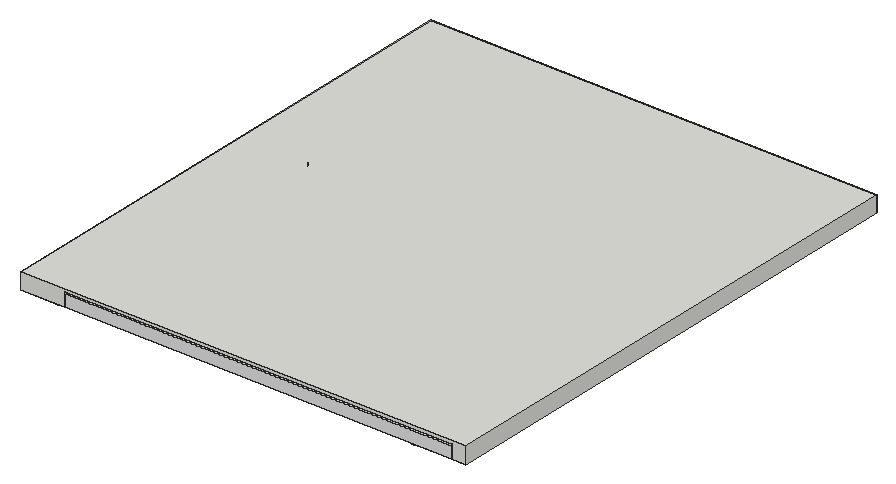
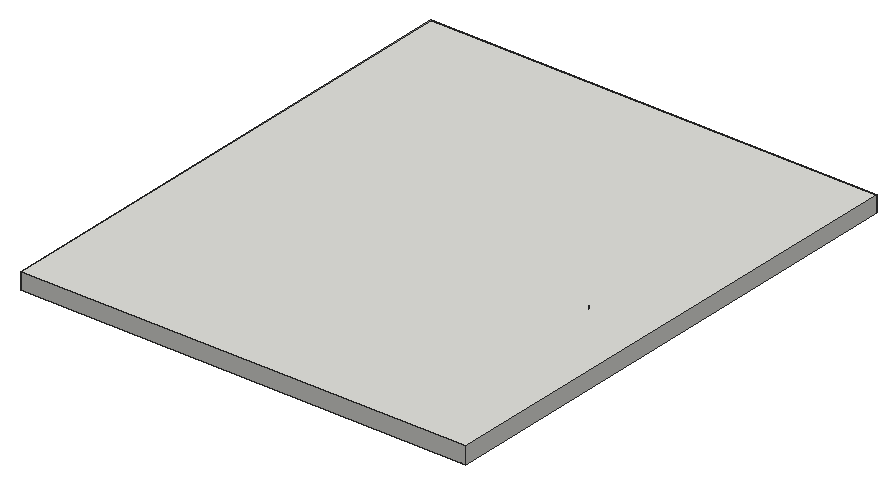
# SketchUp Ruby script. Lengths in inches.
U = 1.inch
M = Sketchup.active_model
def pt(a) = Geom::Point3d.new(a.map { |v| v * U })
def face(e, loops, mat)
  f = e.add_face(loops[0].map { |a| pt(a) })
  loops[1..].each { |l| e.add_face(l.map { |a| pt(a) }).erase! }
  f.material = f.back_material = mat if mat
  f
end
# faces: each face lists its corners as indices into pts; further lists are holes
def faces(e, pts, list, mat = nil) = list.each { |f| face(e, (f[0].is_a?(Array) ? f : [f]).map { |l| l.map { |i| pts[i] } }, mat) }
# xy, xz, yz: faces in a plane at the given z, y or x. An outline is a flat list of corners, or four numbers for a rectangle; further outlines are holes
def ring(l) = l.size == 4 ? [[l[0], l[1]], [l[2], l[1]], [l[2], l[3]], [l[0], l[3]]] : l.each_slice(2).to_a
def flat(e, list, mat, &to3) = list.each { |f| face(e, (f[0].is_a?(Array) ? f : [f]).map { |l| ring(l).map { |u, v| to3.(u, v) } }, mat) }
def xy(e, z, list, mat = nil) = flat(e, list, mat) { |x, y| [x, y, z] }
def xz(e, y, list, mat = nil) = flat(e, list, mat) { |x, z| [x, y, z] }
def yz(e, x, list, mat = nil) = flat(e, list, mat) { |y, z| [x, y, z] }
def lines(e, pts, list) = list.each { |a, b| e.add_line(pt(pts[a]), pt(pts[b])) }
# prism: a flat outline (further loops are holes) pulled along v
def prism(e, loops, v, mat = nil)
  f = face(e, loops, mat); d = Geom::Vector3d.new(v.map { |x| x * U })
  f.pushpull(f.normal.samedirection?(d) ? d.length : -d.length)
end
def box(e, o, s, mat = nil) = prism(e, [[o, [o[0] + s[0], o[1], o[2]], [o[0] + s[0], o[1] + s[1], o[2]], [o[0], o[1] + s[1], o[2]]]], [0, 0, s[2]], mat)
def at(x, y, z, deg = 0) = Geom::Transformation.translation(pt([x, y, z])) * Geom::Transformation.rotation(ORIGIN, Z_AXIS, deg.degrees)
def axes(o, x, y, z) = Geom::Transformation.new([*x, 0, *y, 0, *z, 0, *pt(o).to_a, 1])
def part(name) = M.definitions.add(name)
# library, detail: a bought-in or finely detailed component or shape, given as its bounding box
def library(name, o, s) = part(name).tap { |d| box(d.entities, o, s) }
def detail(e, o, s) = box(e.add_group.entities, o, s)
def put(e, d, t, mat = nil) = e.add_instance(d, t).tap { |i| i.material = mat if mat }
def group(e, t, mat = nil) = e.add_group.tap { |g| g.transformation = t; g.material = mat if mat }.entities
root = M.entities
M.materials.add("[Color M01]").color = [226, 226, 226]
xy(root,206.4375,[[0,0,36.34,0,36.34,513.375,38.125,513.375,38.125,524.91,0,524.91],[36.34,0,38.125,513.375],[38.125,0,45.66,513.375],[441.78,0,441.78,513.375,359.78,513.375,359.78,491.75,319.78,491.75,319.78,502.75,167.66,502.75,167.66,491.75,127.66,491.75,127.66,513.375,38.125,513.375,38.125,524.91,455.6875,524.91,455.6875,0],[400.78,0,409.59,513.375],
  [409.59,0,441.78,513.375]])
xy(root,206.4375,[[[45.66,0,45.66,513.375,127.66,513.375,127.66,491.75,167.66,491.75,167.66,502.75,319.78,502.75,319.78,491.75,359.78,491.75,359.78,513.375,441.78,513.375,441.78,0],[258.62,248.33,273.54,248.91,279.75,249.15,299.95,255.4,317.84,266.68,332.2,282.19,342.05,300.9,346.73,321.52,345.92,342.65,339.66,362.85,328.39,380.74,312.87,395.1,294.16,404.96,273.54,409.64,129.1875,405.59,109.33,403.24,90.75,395.83,74.73,383.86,62.34,368.15,54.45,349.78,51.58,329.99,53.93,310.125,61.34,291.55,73.31,275.52,89.02,263.14,107.39,255.25,127.18,252.38,254.04,249.37],[269.74,224.18,271.3,224.31,272.77,224.83,274.0625,225.72,275.08,226.91,275.75,228.33,276.03,229.87,275.91,231.43,275.38,232.91,274.49,234.2,273.3,235.21,271.88,235.88,270.34,236.16,268.78,236.04,267.31,235.51,266.02,234.625,265,233.43,264.33,232.02,264.05,230.48,264.17,228.91,264.7,227.4375,265.59,226.15,266.78,225.13,268.2,224.46],[270.04,441.17,271.59,441.375,273.04,441.98,274.28,442.93,275.24,444.17,275.84,445.62,276.04,447.17,275.84,448.72,275.24,450.17,274.28,451.41,273.04,452.37,271.59,452.97,270.04,453.17,268.49,452.97,267.04,452.37,265.8,451.41,264.84,450.17,264.24,448.72,264.04,447.17,264.24,445.62,264.84,444.17,265.8,442.93,267.04,441.98,268.49,441.375]],[258.62,248.33,254.04,249.37,273.54,248.91],[265.9375,310.42,261.13,311.05,256.66,312.91,252.8125,315.86,249.86,319.7,248.01,324.18,247.375,328.98,248.01,333.79,249.86,338.26,252.8125,342.11,256.66,345.06,261.13,346.91,265.9375,347.55,270.74,346.91,275.22,345.06,279.0625,342.11,282.01,338.26,283.87,333.79,284.5,328.98,283.87,324.18,282.01,319.7,279.0625,315.86,275.22,312.91,270.74,311.05]],"[Color M01]")
xy(root,208.9375,[[[266.08,284.82,254.65,286.33,244,290.74,234.85,297.76,227.84,306.9,223.42,317.55,221.92,328.98,223.42,340.41,227.84,351.0625,234.85,360.21,244,367.23,254.65,371.64,266.08,373.14,277.51,371.64,288.16,367.23,297.3,360.21,304.32,351.0625,308.73,340.41,310.24,328.98,308.73,317.55,304.32,306.9,297.3,297.76,288.16,290.74,277.51,286.33],[266.08,298.98,273.84,300.01,281.08,303,287.29,307.77,292.06,313.98,295.06,321.22,296.08,328.98,295.06,336.75,292.06,343.98,287.29,350.2,281.08,354.96,273.84,357.96,266.08,358.98,258.3125,357.96,251.08,354.96,244.87,350.2,240.1,343.98,237.1,336.75,236.08,328.98,237.1,321.22,240.1,313.98,244.87,307.77,251.08,303,258.3125,300.01]]],"[Color M01]")
xy(root,209.1875,[[[266.08,298.98,258.3125,300.01,251.08,303,244.87,307.77,240.1,313.98,237.1,321.22,236.08,328.98,237.1,336.75,240.1,343.98,244.87,350.2,251.08,354.96,258.3125,357.96,266.08,358.98,273.84,357.96,281.08,354.96,287.29,350.2,292.06,343.98,295.06,336.75,296.08,328.98,295.06,321.22,292.06,313.98,287.29,307.77,281.08,303,273.84,300.01],[265.9375,310.42,270.74,311.05,275.22,312.91,279.0625,315.86,282.01,319.7,283.87,324.18,284.5,328.98,283.87,333.79,282.01,338.26,279.0625,342.11,275.22,345.06,270.74,346.91,265.9375,347.55,261.13,346.91,256.66,345.06,252.8125,342.11,249.86,338.26,248.01,333.79,247.375,328.98,248.01,324.18,249.86,319.7,252.8125,315.86,256.66,312.91,261.13,311.05]]],"[Color M01]")
xy(root,210,[[269.74,224.18,268.2,224.46,266.78,225.13,265.59,226.15,264.7,227.4375,264.17,228.91,264.05,230.48,264.33,232.02,265,233.43,266.02,234.625,267.31,235.51,268.78,236.04,270.34,236.16,271.88,235.88,273.3,235.21,274.49,234.2,275.38,232.91,275.91,231.43,276.03,229.87,275.75,228.33,275.08,226.91,274.0625,225.72,272.77,224.83,271.3,224.31],[270.04,441.17,268.49,441.375,267.04,441.98,265.8,442.93,264.84,444.17,264.24,445.62,264.04,447.17,264.24,448.72,264.84,450.17,265.8,451.41,267.04,452.37,268.49,452.97,270.04,453.17,271.59,452.97,273.04,452.37,274.28,451.41,275.24,450.17,275.84,448.72,276.04,447.17,275.84,445.62,275.24,444.17,274.28,442.93,273.04,441.98,271.59,441.375]],"[Color M01]")
xy(root,210.125,[[[265.68,267.98,249.9,270.17,235.23,276.36,222.66,286.13,213.05,298.83,207.05,313.58,205.08,329.38,207.26,345.16,213.45,359.83,223.23,372.4,235.93,382.01,250.68,388.01,266.48,389.98,282.25,387.8,296.93,381.61,309.49,371.83,319.11,359.14,325.1,344.38,327.08,328.58,324.89,312.81,318.7,298.14,308.93,285.57,296.23,275.96,281.48,269.96],[266.08,284.82,277.51,286.33,288.16,290.74,297.3,297.76,304.32,306.9,308.73,317.55,310.24,328.98,308.73,340.41,304.32,351.0625,297.3,360.21,288.16,367.23,277.51,371.64,266.08,373.14,254.65,371.64,244,367.23,234.85,360.21,227.84,351.0625,223.42,340.41,221.92,328.98,223.42,317.55,227.84,306.9,234.85,297.76,244,290.74,254.65,286.33]]],"[Color M01]")
xy(root,213,[[[273.54,248.91,254.04,249.37,238,253.01,219.29,262.86,203.77,277.23,194.76,291.52,192.5,295.12,186.24,315.31,185.42,336.44,190.1,357.07,199.96,375.77,214.32,391.29,232.21,402.5625,252.41,408.82,273.54,409.64,294.16,404.96,312.87,395.1,328.39,380.74,339.66,362.85,345.92,342.65,346.73,321.52,342.05,300.9,332.2,282.19,317.84,266.68,299.95,255.4,279.75,249.15],[265.68,267.98,281.48,269.96,296.23,275.96,308.93,285.57,318.7,298.14,324.89,312.81,327.08,328.58,325.1,344.38,319.11,359.14,309.49,371.83,296.93,381.61,282.25,387.8,266.48,389.98,250.68,388.01,235.93,382.01,223.23,372.4,213.45,359.83,207.26,345.16,205.08,329.38,207.05,313.58,213.05,298.83,222.66,286.13,235.23,276.36,249.9,270.17]],[124.34,305.51,118.27,307.06,112.8125,310.13,108.33,314.51,105.14,319.9,103.45,325.93,103.38,332.2,104.93,338.27,108.01,343.73,112.39,348.21,117.78,351.4,123.81,353.09,130.07,353.16,136.14,351.61,141.6,348.54,146.08,344.16,149.28,338.77,150.97,332.73,151.04,326.47,149.48,320.4,146.41,314.9375,142.03,310.46,136.64,307.27,130.61,305.58]],"[Color M01]")
xy(root,216.0625,[[[124.34,305.51,130.61,305.58,136.64,307.27,142.03,310.46,146.41,314.9375,149.48,320.4,151.04,326.47,150.97,332.73,149.28,338.77,146.08,344.16,141.6,348.54,136.14,351.61,130.07,353.16,123.81,353.09,117.78,351.4,112.39,348.21,108.01,343.73,104.93,338.27,103.38,332.2,103.45,325.93,105.14,319.9,108.33,314.51,112.8125,310.13,118.27,307.06],[128.1875,310.48,123.4,311.11,118.9375,312.96,115.1,315.9,112.16,319.73,110.32,324.2,109.6875,328.98,110.32,333.77,112.16,338.23,115.1,342.07,118.9375,345.01,123.4,346.85,128.1875,347.48,132.97,346.85,137.4375,345.01,141.27,342.07,144.21,338.23,146.06,333.77,146.6875,328.98,146.06,324.2,144.21,319.73,141.27,315.9,137.4375,312.96,132.97,311.11]]],"[Color M01]")
xy(root,216.4375,[[[254.04,249.37,127.18,252.38,107.39,255.25,89.02,263.14,73.31,275.52,61.34,291.55,53.93,310.125,51.58,329.99,54.45,349.78,62.34,368.15,74.73,383.86,90.75,395.83,109.33,403.24,129.1875,405.59,273.54,409.64,252.41,408.82,232.21,402.5625,214.32,391.29,199.96,375.77,190.1,357.07,185.42,336.44,186.24,315.31,192.5,295.12,194.76,291.52,203.77,277.23,219.29,262.86,238,253.01],[128.1875,310.48,132.97,311.11,137.4375,312.96,141.27,315.9,144.21,319.73,146.06,324.2,146.6875,328.98,146.06,333.77,144.21,338.23,141.27,342.07,137.4375,345.01,132.97,346.85,128.1875,347.48,123.4,346.85,118.9375,345.01,115.1,342.07,112.16,338.23,110.32,333.77,109.6875,328.98,110.32,324.2,112.16,319.73,115.1,315.9,118.9375,312.96,123.4,311.11]]],"[Color M01]")
xy(root,218.875,[[45.66,0,441.78,0,441.78,513.375,359.78,513.375,359.78,491.75,319.78,491.75,319.78,502.75,167.66,502.75,167.66,491.75,127.66,491.75,127.66,513.375,45.66,513.375]],"[Color M01]")
xy(root,220.25,[[45.66,0,45.66,513.375,127.66,513.375,127.66,491.75,167.66,491.75,167.66,502.75,319.78,502.75,319.78,491.75,359.78,491.75,359.78,513.375,441.78,513.375,441.78,0]])
xy(root,223.0625,[[0,0,455.6875,524.91]])
xz(root,0,[[0,206.4375,45.66,206.4375,45.66,220.25,441.78,220.25,441.78,206.4375,455.6875,206.4375,455.6875,223.0625,0,223.0625]])
xz(root,0,[[45.66,206.4375,441.78,218.875]],"[Color M01]")
xz(root,491.75,[[127.66,206.4375,167.66,220.25],[319.78,206.4375,359.78,220.25]])
xz(root,491.75,[[127.66,206.4375,167.66,218.875],[319.78,206.4375,359.78,218.875]],"[Color M01]")
xz(root,502.75,[[167.66,206.4375,319.78,220.25]])
xz(root,502.75,[[167.66,206.4375,319.78,218.875]],"[Color M01]")
xz(root,513.375,[[45.66,206.4375,127.66,220.25],[359.78,206.4375,441.78,220.25]])
xz(root,513.375,[[45.66,206.4375,127.66,218.875],[359.78,206.4375,441.78,218.875]],"[Color M01]")
xz(root,524.91,[[0,206.4375,455.6875,223.0625]])
yz(root,0,[[0,206.4375,524.91,223.0625]])
yz(root,45.66,[[0,206.4375,513.375,220.25]])
yz(root,45.66,[[0,206.4375,513.375,218.875]],"[Color M01]")
yz(root,127.66,[[491.75,206.4375,513.375,220.25]])
yz(root,127.66,[[491.75,206.4375,513.375,218.875]],"[Color M01]")
yz(root,167.66,[[491.75,206.4375,502.75,220.25]])
yz(root,167.66,[[491.75,206.4375,502.75,218.875]],"[Color M01]")
yz(root,319.78,[[491.75,206.4375,502.75,220.25]])
yz(root,319.78,[[491.75,206.4375,502.75,218.875]],"[Color M01]")
yz(root,359.78,[[491.75,206.4375,513.375,220.25]])
yz(root,359.78,[[491.75,206.4375,513.375,218.875]],"[Color M01]")
yz(root,441.78,[[0,206.4375,513.375,220.25]])
yz(root,441.78,[[0,206.4375,513.375,218.875]],"[Color M01]")
yz(root,455.6875,[[0,206.4375,524.91,223.0625]])
p = [[401.6875,513.375,206.01],[402.57,513.375,205.53],[402.57,0,205.53],[401.6875,0,206.01],[400.78,513.375,206.4375],[400.78,0,206.4375],
  [269.74,224.18,206.4375],[268.2,224.46,206.4375],[268.2,224.46,210],[269.74,224.18,210],[271.3,224.31,206.4375],[271.3,224.31,210],
  [272.77,224.83,206.4375],[272.77,224.83,210],[266.78,225.13,206.4375],[266.78,225.13,210],[274.0625,225.72,206.4375],[274.0625,225.72,210],
  [265.59,226.15,206.4375],[265.59,226.15,210],[275.08,226.91,206.4375],[275.08,226.91,210],[264.7,227.4375,206.4375],[264.7,227.4375,210],
  [275.75,228.33,206.4375],[275.75,228.33,210],[264.17,228.91,206.4375],[264.17,228.91,210],[276.03,229.87,206.4375],[276.03,229.87,210],
  [264.05,230.48,206.4375],[264.05,230.48,210],[275.91,231.43,206.4375],[275.91,231.43,210],[264.33,232.02,206.4375],[264.33,232.02,210],
  [275.38,232.91,206.4375],[275.38,232.91,210],[265,233.43,206.4375],[265,233.43,210],[274.49,234.2,206.4375],[274.49,234.2,210],
  [266.02,234.625,206.4375],[266.02,234.625,210],[273.3,235.21,206.4375],[273.3,235.21,210],[267.31,235.51,206.4375],[267.31,235.51,210],
  [271.88,235.88,206.4375],[271.88,235.88,210],[268.78,236.04,206.4375],[268.78,236.04,210],[270.34,236.16,206.4375],[270.34,236.16,210],
  [273.54,248.91,206.4375],[254.04,249.37,206.4375],[254.04,249.37,213],[273.54,248.91,213],[279.75,249.15,206.4375],[279.75,249.15,213],
  [299.95,255.4,206.4375],[299.95,255.4,213],[127.18,252.38,206.4375],[127.18,252.38,216.4375],[254.04,249.37,216.4375],[107.39,255.25,206.4375],
  [107.39,255.25,216.4375],[89.02,263.14,206.4375],[89.02,263.14,216.4375],[317.84,266.68,206.4375],[317.84,266.68,213],[73.31,275.52,206.4375],
  [73.31,275.52,216.4375],[332.2,282.19,206.4375],[332.2,282.19,213],[61.34,291.55,206.4375],[61.34,291.55,216.4375],[342.05,300.9,206.4375],
  [342.05,300.9,213],[53.93,310.125,206.4375],[53.93,310.125,216.4375],[346.73,321.52,206.4375],[346.73,321.52,213],[51.58,329.99,206.4375],
  [51.58,329.99,216.4375],[261.13,311.05,206.4375],[265.9375,310.42,206.4375],[265.9375,310.42,209.1875],[261.13,311.05,209.1875],[270.74,311.05,206.4375],
  [270.74,311.05,209.1875],[256.66,312.91,206.4375],[256.66,312.91,209.1875],[275.22,312.91,206.4375],[275.22,312.91,209.1875],[252.8125,315.86,206.4375],
  [252.8125,315.86,209.1875],[279.0625,315.86,206.4375],[279.0625,315.86,209.1875],[249.86,319.7,206.4375],[249.86,319.7,209.1875],[282.01,319.7,206.4375],
  [282.01,319.7,209.1875],[248.01,324.18,206.4375],[248.01,324.18,209.1875],[283.87,324.18,206.4375],[283.87,324.18,209.1875],[345.92,342.65,206.4375],
  [345.92,342.65,213],[247.375,328.98,206.4375],[247.375,328.98,209.1875],[284.5,328.98,206.4375],[284.5,328.98,209.1875],[248.01,333.79,206.4375],
  [248.01,333.79,209.1875],[283.87,333.79,206.4375],[283.87,333.79,209.1875],[54.45,349.78,206.4375],[54.45,349.78,216.4375],[249.86,338.26,206.4375],
  [249.86,338.26,209.1875],[282.01,338.26,206.4375],[282.01,338.26,209.1875],[252.8125,342.11,206.4375],[252.8125,342.11,209.1875],[279.0625,342.11,206.4375],
  [279.0625,342.11,209.1875],[256.66,345.06,206.4375],[256.66,345.06,209.1875],[275.22,345.06,206.4375],[275.22,345.06,209.1875],[339.66,362.85,206.4375],
  [339.66,362.85,213],[261.13,346.91,206.4375],[261.13,346.91,209.1875],[270.74,346.91,206.4375],[270.74,346.91,209.1875],[265.9375,347.55,206.4375],
  [265.9375,347.55,209.1875],[62.34,368.15,206.4375],[62.34,368.15,216.4375],[328.39,380.74,206.4375],[328.39,380.74,213],[74.73,383.86,206.4375],
  [74.73,383.86,216.4375],[312.87,395.1,206.4375],[312.87,395.1,213],[90.75,395.83,206.4375],[90.75,395.83,216.4375],[294.16,404.96,206.4375],
  [294.16,404.96,213],[109.33,403.24,206.4375],[109.33,403.24,216.4375],[129.1875,405.59,206.4375],[129.1875,405.59,216.4375],[273.54,409.64,206.4375],
  [273.54,409.64,213],[273.54,409.64,216.4375],[270.04,441.17,206.4375],[268.49,441.375,206.4375],[268.49,441.375,210],[270.04,441.17,210],
  [271.59,441.375,206.4375],[271.59,441.375,210],[267.04,441.98,206.4375],[267.04,441.98,210],[273.04,441.98,206.4375],[273.04,441.98,210],
  [265.8,442.93,206.4375],[265.8,442.93,210],[274.28,442.93,206.4375],[274.28,442.93,210],[264.84,444.17,206.4375],[264.84,444.17,210],
  [275.24,444.17,206.4375],[275.24,444.17,210],[264.24,445.62,206.4375],[264.24,445.62,210],[275.84,445.62,206.4375],[275.84,445.62,210],
  [264.04,447.17,206.4375],[264.04,447.17,210],[276.04,447.17,206.4375],[276.04,447.17,210],[264.24,448.72,206.4375],[264.24,448.72,210],
  [275.84,448.72,206.4375],[275.84,448.72,210],[264.84,450.17,206.4375],[264.84,450.17,210],[275.24,450.17,206.4375],[275.24,450.17,210],
  [265.8,451.41,206.4375],[265.8,451.41,210],[274.28,451.41,206.4375],[274.28,451.41,210],[267.04,452.37,206.4375],[267.04,452.37,210],
  [273.04,452.37,206.4375],[273.04,452.37,210],[268.49,452.97,206.4375],[268.49,452.97,210],[271.59,452.97,206.4375],[271.59,452.97,210],
  [270.04,453.17,206.4375],[270.04,453.17,210],[254.65,286.33,210.125],[254.65,286.33,208.9375],[266.08,284.82,208.9375],[266.08,284.82,210.125],
  [277.51,286.33,208.9375],[277.51,286.33,210.125],[244,290.74,210.125],[244,290.74,208.9375],[288.16,290.74,208.9375],[288.16,290.74,210.125],
  [234.85,297.76,210.125],[234.85,297.76,208.9375],[297.3,297.76,208.9375],[297.3,297.76,210.125],[227.84,306.9,210.125],[227.84,306.9,208.9375],
  [304.32,306.9,208.9375],[304.32,306.9,210.125],[258.3125,300.01,208.9375],[258.3125,300.01,209.1875],[266.08,298.98,209.1875],[266.08,298.98,208.9375],
  [273.84,300.01,209.1875],[273.84,300.01,208.9375],[251.08,303,208.9375],[251.08,303,209.1875],[281.08,303,209.1875],[281.08,303,208.9375],
  [244.87,307.77,208.9375],[244.87,307.77,209.1875],[287.29,307.77,209.1875],[287.29,307.77,208.9375],[223.42,317.55,210.125],[223.42,317.55,208.9375],
  [308.73,317.55,208.9375],[308.73,317.55,210.125],[240.1,313.98,208.9375],[240.1,313.98,209.1875],[292.06,313.98,209.1875],[292.06,313.98,208.9375],
  [237.1,321.22,208.9375],[237.1,321.22,209.1875],[295.06,321.22,209.1875],[295.06,321.22,208.9375],[221.92,328.98,210.125],[221.92,328.98,208.9375],
  [310.24,328.98,208.9375],[310.24,328.98,210.125],[236.08,328.98,208.9375],[236.08,328.98,209.1875],[296.08,328.98,209.1875],[296.08,328.98,208.9375],
  [223.42,340.41,210.125],[223.42,340.41,208.9375],[237.1,336.75,208.9375],[237.1,336.75,209.1875],[295.06,336.75,209.1875],[295.06,336.75,208.9375],
  [308.73,340.41,208.9375],[308.73,340.41,210.125],[240.1,343.98,208.9375],[240.1,343.98,209.1875],[292.06,343.98,209.1875],[292.06,343.98,208.9375],
  [227.84,351.0625,210.125],[227.84,351.0625,208.9375],[304.32,351.0625,208.9375],[304.32,351.0625,210.125],[244.87,350.2,208.9375],[244.87,350.2,209.1875],
  [287.29,350.2,209.1875],[287.29,350.2,208.9375],[251.08,354.96,208.9375],[251.08,354.96,209.1875],[281.08,354.96,209.1875],[281.08,354.96,208.9375],
  [234.85,360.21,210.125],[234.85,360.21,208.9375],[297.3,360.21,208.9375],[297.3,360.21,210.125],[258.3125,357.96,208.9375],[258.3125,357.96,209.1875],
  [273.84,357.96,209.1875],[273.84,357.96,208.9375],[266.08,358.98,208.9375],[266.08,358.98,209.1875],[244,367.23,210.125],[244,367.23,208.9375],
  [288.16,367.23,208.9375],[288.16,367.23,210.125],[254.65,371.64,210.125],[254.65,371.64,208.9375],[277.51,371.64,208.9375],[277.51,371.64,210.125],
  [266.08,373.14,210.125],[266.08,373.14,208.9375],[249.9,270.17,213],[249.9,270.17,210.125],[265.68,267.98,210.125],[265.68,267.98,213],
  [281.48,269.96,210.125],[281.48,269.96,213],[296.23,275.96,210.125],[296.23,275.96,213],[235.23,276.36,213],[235.23,276.36,210.125],
  [308.93,285.57,210.125],[308.93,285.57,213],[222.66,286.13,213],[222.66,286.13,210.125],[318.7,298.14,210.125],[318.7,298.14,213],
  [213.05,298.83,213],[213.05,298.83,210.125],[324.89,312.81,210.125],[324.89,312.81,213],[207.05,313.58,213],[207.05,313.58,210.125],
  [327.08,328.58,210.125],[327.08,328.58,213],[205.08,329.38,213],[205.08,329.38,210.125],[325.1,344.38,210.125],[325.1,344.38,213],
  [207.26,345.16,213],[207.26,345.16,210.125],[319.11,359.14,210.125],[319.11,359.14,213],[213.45,359.83,213],[213.45,359.83,210.125],
  [309.49,371.83,210.125],[309.49,371.83,213],[223.23,372.4,213],[223.23,372.4,210.125],[296.93,381.61,210.125],[296.93,381.61,213],
  [235.93,382.01,213],[235.93,382.01,210.125],[282.25,387.8,210.125],[282.25,387.8,213],[250.68,388.01,213],[250.68,388.01,210.125],
  [266.48,389.98,210.125],[266.48,389.98,213],[238,253.01,216.4375],[238,253.01,213],[219.29,262.86,216.4375],[219.29,262.86,213],
  [203.77,277.23,216.4375],[203.77,277.23,213],[194.76,291.52,216.4375],[194.76,291.52,213],[192.5,295.12,216.4375],[192.5,295.12,213],
  [186.24,315.31,216.4375],[186.24,315.31,213],[118.27,307.06,213],[124.34,305.51,213],[124.34,305.51,216.0625],[118.27,307.06,216.0625],
  [130.61,305.58,213],[130.61,305.58,216.0625],[136.64,307.27,213],[136.64,307.27,216.0625],[112.8125,310.13,213],[112.8125,310.13,216.0625],
  [142.03,310.46,213],[142.03,310.46,216.0625],[108.33,314.51,213],[108.33,314.51,216.0625],[146.41,314.9375,213],[146.41,314.9375,216.0625],
  [105.14,319.9,213],[105.14,319.9,216.0625],[149.48,320.4,213],[149.48,320.4,216.0625],[185.42,336.44,216.4375],[185.42,336.44,213],
  [103.45,325.93,213],[103.45,325.93,216.0625],[151.04,326.47,213],[151.04,326.47,216.0625],[103.38,332.2,213],[103.38,332.2,216.0625],
  [150.97,332.73,213],[150.97,332.73,216.0625],[104.93,338.27,213],[104.93,338.27,216.0625],[149.28,338.77,213],[149.28,338.77,216.0625],
  [190.1,357.07,216.4375],[190.1,357.07,213],[108.01,343.73,213],[108.01,343.73,216.0625],[146.08,344.16,213],[146.08,344.16,216.0625],
  [112.39,348.21,213],[112.39,348.21,216.0625],[141.6,348.54,213],[141.6,348.54,216.0625],[117.78,351.4,213],[117.78,351.4,216.0625],
  [136.14,351.61,213],[136.14,351.61,216.0625],[123.81,353.09,213],[123.81,353.09,216.0625],[130.07,353.16,213],[130.07,353.16,216.0625],
  [195.03,366.42,216.4375],[195.03,366.42,213],[199.96,375.77,216.4375],[199.96,375.77,213],[214.32,391.29,216.4375],[214.32,391.29,213],
  [232.21,402.5625,216.4375],[232.21,402.5625,213],[252.41,408.82,216.4375],[252.41,408.82,213],[123.4,311.11,216.4375],[123.4,311.11,216.0625],
  [128.1875,310.48,216.0625],[128.1875,310.48,216.4375],[132.97,311.11,216.0625],[132.97,311.11,216.4375],[118.9375,312.96,216.4375],[118.9375,312.96,216.0625],
  [137.4375,312.96,216.0625],[137.4375,312.96,216.4375],[115.1,315.9,216.4375],[115.1,315.9,216.0625],[141.27,315.9,216.0625],[141.27,315.9,216.4375],
  [112.16,319.73,216.4375],[112.16,319.73,216.0625],[144.21,319.73,216.0625],[144.21,319.73,216.4375],[110.32,324.2,216.4375],[110.32,324.2,216.0625],
  [146.06,324.2,216.0625],[146.06,324.2,216.4375],[109.6875,328.98,216.4375],[109.6875,328.98,216.0625],[146.6875,328.98,216.0625],[146.6875,328.98,216.4375],
  [110.32,333.77,216.4375],[110.32,333.77,216.0625],[146.06,333.77,216.0625],[146.06,333.77,216.4375],[112.16,338.23,216.4375],[112.16,338.23,216.0625],
  [144.21,338.23,216.0625],[144.21,338.23,216.4375],[115.1,342.07,216.4375],[115.1,342.07,216.0625],[141.27,342.07,216.0625],[141.27,342.07,216.4375],
  [118.9375,345.01,216.4375],[118.9375,345.01,216.0625],[137.4375,345.01,216.0625],[137.4375,345.01,216.4375],[123.4,346.85,216.4375],[123.4,346.85,216.0625],
  [132.97,346.85,216.0625],[132.97,346.85,216.4375],[128.1875,347.48,216.4375],[128.1875,347.48,216.0625]]
faces(root,p,[[0,1,2,3],[4,0,3,5]])
faces(root,p,[[6,7,8,9],[10,6,9,11],[12,10,11,13],[7,14,15,8],[16,12,13,17],[14,18,19,15],[20,16,17,21],[18,22,23,19],
  [24,20,21,25],[22,26,27,23],[28,24,25,29],[26,30,31,27],[32,28,29,33],[30,34,35,31],[36,32,33,37],[34,38,39,35],
  [40,36,37,41],[38,42,43,39],[44,40,41,45],[42,46,47,43],[48,44,45,49],[46,50,51,47],[52,48,49,53],[50,52,53,51],
  [54,55,56,57],[58,54,57,59],[60,58,59,61],[55,62,63,64,56],[62,65,66,63],[65,67,68,66],[69,60,61,70],[67,71,72,68],
  [73,69,70,74],[71,75,76,72],[77,73,74,78],[75,79,80,76],[81,77,78,82],[79,83,84,80],[85,86,87,88],[86,89,90,87],
  [91,85,88,92],[89,93,94,90],[95,91,92,96],[93,97,98,94],[99,95,96,100],[97,101,102,98],[103,99,100,104],[101,105,106,102],
  [107,81,82,108],[109,103,104,110],[105,111,112,106],[113,109,110,114],[111,115,116,112],[83,117,118,84],[119,113,114,120],[115,121,122,116],
  [123,119,120,124],[121,125,126,122],[127,123,124,128],[125,129,130,126],[131,107,108,132],[133,127,128,134],[129,135,136,130],[137,133,134,138],
  [135,137,138,136],[117,139,140,118],[141,131,132,142],[139,143,144,140],[145,141,142,146],[143,147,148,144],[149,145,146,150],[147,151,152,148],
  [151,153,154,152],[155,149,150,156],[153,155,156,157,154],[158,159,160,161],[162,158,161,163],[159,164,165,160],[166,162,163,167],[164,168,169,165],
  [170,166,167,171],[168,172,173,169],[174,170,171,175],[172,176,177,173],[178,174,175,179],[176,180,181,177],[182,178,179,183],[180,184,185,181],
  [186,182,183,187],[184,188,189,185],[190,186,187,191],[188,192,193,189],[194,190,191,195],[192,196,197,193],[198,194,195,199],[196,200,201,197],
  [202,198,199,203],[200,204,205,201],[204,202,203,205],[206,207,208,209],[209,208,210,211],[212,213,207,206],[211,210,214,215],[216,217,213,212],
  [215,214,218,219],[220,221,217,216],[219,218,222,223],[224,225,226,227],[227,226,228,229],[230,231,225,224],[229,228,232,233],[234,235,231,230],
  [233,232,236,237],[238,239,221,220],[223,222,240,241],[242,243,235,234],[237,236,244,245],[246,247,243,242],[245,244,248,249],[250,251,239,238],
  [241,240,252,253],[254,255,247,246],[249,248,256,257],[258,259,251,250],[260,261,255,254],[257,256,262,263],[253,252,264,265],[266,267,261,260],
  [263,262,268,269],[270,271,259,258],[265,264,272,273],[274,275,267,266],[269,268,276,277],[278,279,275,274],[277,276,280,281],[282,283,271,270],
  [273,272,284,285],[286,287,279,278],[281,280,288,289],[290,291,287,286],[289,288,291,290],[292,293,283,282],[285,284,294,295],[296,297,293,292],
  [295,294,298,299],[300,301,297,296],[299,298,301,300],[302,303,304,305],[305,304,306,307],[307,306,308,309],[310,311,303,302],[309,308,312,313],
  [314,315,311,310],[313,312,316,317],[318,319,315,314],[317,316,320,321],[322,323,319,318],[321,320,324,325],[326,327,323,322],[325,324,328,329],
  [330,331,327,326],[329,328,332,333],[334,335,331,330],[333,332,336,337],[338,339,335,334],[337,336,340,341],[342,343,339,338],[341,340,344,345],
  [346,347,343,342],[345,344,348,349],[349,348,347,346],[350,351,56,64],[352,353,351,350],[354,355,353,352],[356,357,355,354],[358,359,357,356],
  [360,361,359,358],[362,363,364,365],[363,366,367,364],[366,368,369,367],[370,362,365,371],[368,372,373,369],[374,370,371,375],[372,376,377,373],
  [378,374,375,379],[376,380,381,377],[382,383,361,360],[384,378,379,385],[380,386,387,381],[388,384,385,389],[386,390,391,387],[392,388,389,393],
  [390,394,395,391],[396,397,383,382],[398,392,393,399],[394,400,401,395],[402,398,399,403],[400,404,405,401],[406,402,403,407],[404,408,409,405],
  [410,406,407,411],[408,412,413,409],[412,410,411,413],[414,415,397,396],[416,417,415,414],[418,419,417,416],[420,421,419,418],[422,423,421,420],
  [157,156,423,422],[424,425,426,427],[427,426,428,429],[430,431,425,424],[429,428,432,433],[434,435,431,430],[433,432,436,437],[438,439,435,434],
  [437,436,440,441],[442,443,439,438],[441,440,444,445],[446,447,443,442],[445,444,448,449],[450,451,447,446],[449,448,452,453],[454,455,451,450],
  [453,452,456,457],[458,459,455,454],[457,456,460,461],[462,463,459,458],[461,460,464,465],[466,467,463,462],[465,464,468,469],[470,471,467,466],
  [469,468,471,470]],"[Color M01]")
